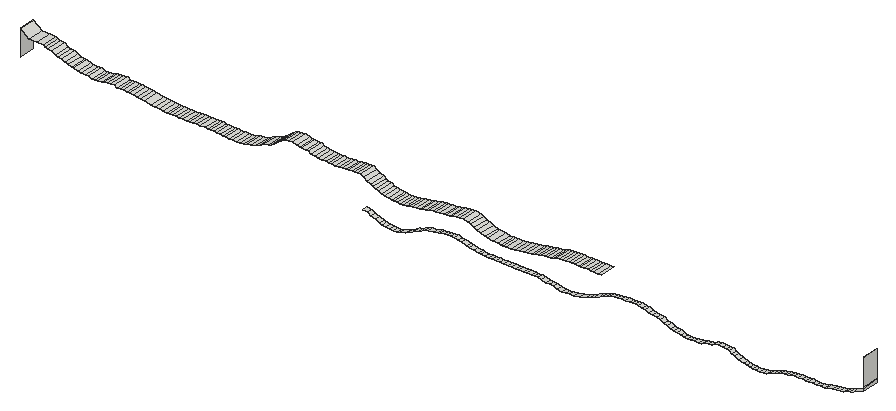
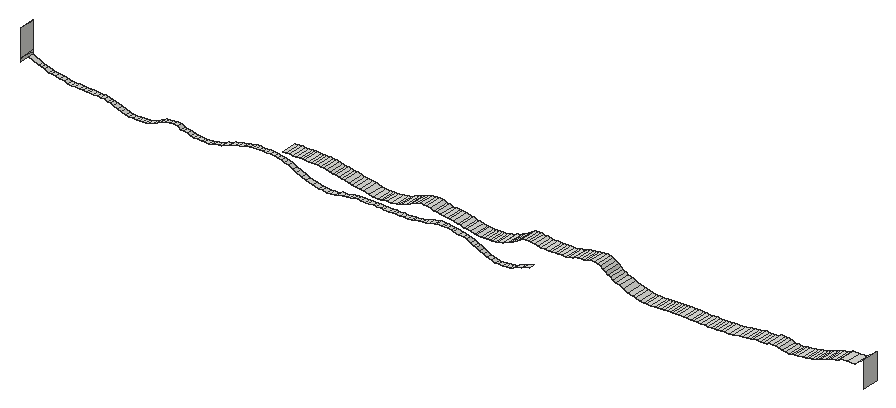
# SketchUp Ruby script. Lengths in inches.
U = 1.inch
M = Sketchup.active_model
def pt(a) = Geom::Point3d.new(a.map { |v| v * U })
def face(e, loops, mat)
  f = e.add_face(loops[0].map { |a| pt(a) })
  loops[1..].each { |l| e.add_face(l.map { |a| pt(a) }).erase! }
  f.material = f.back_material = mat if mat
  f
end
# faces: each face lists its corners as indices into pts; further lists are holes
def faces(e, pts, list, mat = nil) = list.each { |f| face(e, (f[0].is_a?(Array) ? f : [f]).map { |l| l.map { |i| pts[i] } }, mat) }
# xy, xz, yz: faces in a plane at the given z, y or x. An outline is a flat list of corners, or four numbers for a rectangle; further outlines are holes
def ring(l) = l.size == 4 ? [[l[0], l[1]], [l[2], l[1]], [l[2], l[3]], [l[0], l[3]]] : l.each_slice(2).to_a
def flat(e, list, mat, &to3) = list.each { |f| face(e, (f[0].is_a?(Array) ? f : [f]).map { |l| ring(l).map { |u, v| to3.(u, v) } }, mat) }
def xy(e, z, list, mat = nil) = flat(e, list, mat) { |x, y| [x, y, z] }
def xz(e, y, list, mat = nil) = flat(e, list, mat) { |x, z| [x, y, z] }
def yz(e, x, list, mat = nil) = flat(e, list, mat) { |y, z| [x, y, z] }
def lines(e, pts, list) = list.each { |a, b| e.add_line(pt(pts[a]), pt(pts[b])) }
# prism: a flat outline (further loops are holes) pulled along v
def prism(e, loops, v, mat = nil)
  f = face(e, loops, mat); d = Geom::Vector3d.new(v.map { |x| x * U })
  f.pushpull(f.normal.samedirection?(d) ? d.length : -d.length)
end
def box(e, o, s, mat = nil) = prism(e, [[o, [o[0] + s[0], o[1], o[2]], [o[0] + s[0], o[1] + s[1], o[2]], [o[0], o[1] + s[1], o[2]]]], [0, 0, s[2]], mat)
def at(x, y, z, deg = 0) = Geom::Transformation.translation(pt([x, y, z])) * Geom::Transformation.rotation(ORIGIN, Z_AXIS, deg.degrees)
def axes(o, x, y, z) = Geom::Transformation.new([*x, 0, *y, 0, *z, 0, *pt(o).to_a, 1])
def part(name) = M.definitions.add(name)
# library, detail: a bought-in or finely detailed component or shape, given as its bounding box
def library(name, o, s) = part(name).tap { |d| box(d.entities, o, s) }
def detail(e, o, s) = box(e.add_group.entities, o, s)
def put(e, d, t, mat = nil) = e.add_instance(d, t).tap { |i| i.material = mat if mat }
def group(e, t, mat = nil) = e.add_group.tap { |g| g.transformation = t; g.material = mat if mat }.entities
root = M.entities
xy(root,238.18,[[376.03,2401.37,376.71,2402.3]])
xy(root,238.62,[[342.56,2401.37,343.33,2402.3],[343.33,2401.37,343.96,2402.3],[343.96,2401.37,344.72,2402.3],[344.72,2401.37,345.34,2402.3],[345.34,2401.37,346.19,2402.3],
  [346.19,2401.37,346.83,2402.3],[346.83,2401.37,347.45,2402.3]])
xy(root,238.625,[[341.14,2401.37,342,2402.3]])
xy(root,238.89,[[396.95,2401.37,397.63,2402.3]])
xy(root,238.9,[[398.39,2401.37,399.01,2402.3],[399.01,2401.37,399.78,2402.3]])
xy(root,240.43,[[365.23,2401.37,365.8,2402.3]])
xy(root,241.68,[[283.28,2401.37,283.87,2404.3]])
xy(root,241.75,[[285.63,2401.37,286.5,2404.3],[286.5,2401.37,287.12,2404.3],[287.12,2401.37,287.63,2404.3]])
xy(root,243.05,[[358.29,2401.37,358.97,2404.3]])
xy(root,243.07,[[356.4375,2401.37,357.02,2404.3]])
xy(root,243.09,[[353.125,2401.37,353.65,2404.3],[353.65,2401.37,354.17,2404.3],[354.17,2401.37,354.83,2404.3],[354.83,2401.37,355.28,2404.3]])
yz(root,252.84,[[2401.37,241.52,2404.3,246.2]])
yz(root,406.85,[[2401.37,240.89,2401.37,241.29,2404.3,241.52,2404.3,240.89],[2401.37,241.29,2404.3,241.52,2401.37,241.52],[2401.37,241.52,2401.37,246.27,2402.0625,246.36,2404.3,246.43,2404.3,241.52],[2401.37,246.27,2401.37,246.43,2404.3,246.43,2402.0625,246.36]])
p = [[319.64,2401.37,237.11],[319.64,2402.3,237.11],[320.4,2402.3,237.04],[320.4,2401.37,237.04],[321.09,2402.3,237.01],[321.09,2401.37,237.01],
  [321.7,2402.3,236.98],[321.7,2401.37,236.98],[322.38,2402.3,237.22],[322.38,2401.37,237.22],[318.95,2401.37,237.2],[318.95,2402.3,237.2],
  [318.42,2401.37,237.33],[318.42,2402.3,237.33],[323.23,2402.3,237.43],[323.23,2401.37,237.43],[317.75,2401.37,237.68],[317.75,2402.3,237.68],
  [323.85,2402.3,237.74],[323.85,2401.37,237.74],[386.68,2401.37,237.45],[386.68,2402.3,237.45],[387.25,2402.3,237.42],[387.25,2401.37,237.42],
  [387.98,2402.3,237.4],[387.98,2401.37,237.4],[388.66,2402.3,237.47],[388.66,2401.37,237.47],[385.49,2401.37,237.59],[385.49,2402.3,237.59],
  [386.09,2402.3,237.51],[386.09,2401.37,237.51],[389.26,2402.3,237.5625],[389.26,2401.37,237.5625],[384.95,2401.37,237.71],[384.95,2402.3,237.71],
  [389.95,2402.3,237.84],[389.95,2401.37,237.84],[316.8125,2401.37,237.96],[316.8125,2402.3,237.96],[324.55,2402.3,238.02],[324.55,2401.37,238.02],
  [351.69,2401.37,237.79],[351.69,2402.3,237.79],[352.4,2402.3,237.74],[352.4,2401.37,237.74],[353.27,2402.3,237.87],[353.27,2401.37,237.87],
  [384.12,2401.37,238],[384.12,2402.3,238],[350.92,2401.37,237.86],[350.92,2402.3,237.86],[390.63,2402.3,238.08],[390.63,2401.37,238.08],
  [350.29,2401.37,238.15],[350.29,2402.3,238.15],[353.92,2402.3,237.88],[353.92,2401.37,237.88],[355.04,2402.3,238.14],[355.04,2401.37,238.14],
  [316.25,2401.37,238.28],[316.25,2402.3,238.28],[324.99,2402.3,238.375],[324.99,2401.37,238.375],[383.41,2401.37,238.33],[383.41,2402.3,238.33],
  [349.52,2401.37,238.19],[349.52,2402.3,238.19],[356.26,2402.3,238.46],[356.26,2401.37,238.46],[374.01,2401.37,238.19],[374.01,2402.3,238.19],
  [374.83,2402.3,238.15],[374.83,2401.37,238.15],[375.36,2402.3,238.11],[375.36,2401.37,238.11],[376.03,2402.3,238.18],[376.03,2401.37,238.18],
  [391.32,2402.3,238.33],[391.32,2401.37,238.33],[348.9,2401.37,238.25],[348.9,2402.3,238.25],[373.4375,2401.37,238.26],[373.4375,2402.3,238.26],
  [376.71,2401.37,238.18],[376.71,2402.3,238.18],[377.39,2402.3,238.27],[377.39,2401.37,238.27],[315.47,2401.37,238.43],[315.47,2402.3,238.43],
  [348.14,2401.37,238.45],[348.14,2402.3,238.45],[372.87,2401.37,238.48],[372.87,2402.3,238.48],[377.91,2402.3,238.55],[377.91,2401.37,238.55],
  [382.86,2401.37,238.57],[382.86,2402.3,238.57],[391.85,2402.3,238.51],[391.85,2401.37,238.51],[325.55,2402.3,238.51],[325.55,2401.37,238.51],
  [326.1875,2402.3,238.76],[326.1875,2401.37,238.76],[347.45,2401.37,238.62],[347.45,2402.3,238.62],[357.01,2402.3,238.72],[357.01,2401.37,238.72],
  [372.21,2401.37,238.56],[372.21,2402.3,238.56],[378.57,2402.3,238.61],[378.57,2401.37,238.61],[392.42,2402.3,238.6],[392.42,2401.37,238.6],
  [338.38,2401.37,238.66],[338.38,2402.3,238.66],[339.05,2402.3,238.65],[339.05,2401.37,238.65],[339.83,2402.3,238.64],[339.83,2401.37,238.64],
  [340.45,2402.3,238.63],[340.45,2401.37,238.63],[341.14,2402.3,238.625],[341.14,2401.37,238.625],[342,2401.37,238.625],[342,2402.3,238.625],
  [342.56,2402.3,238.62],[342.56,2401.37,238.62],[371.64,2401.37,238.67],[371.64,2402.3,238.67],[379.16,2402.3,238.66],[379.16,2401.37,238.66],
  [382.36,2401.37,238.86],[382.36,2402.3,238.86],[393.08,2402.3,238.74],[393.08,2401.37,238.74],[336.54,2401.37,238.78],[336.54,2402.3,238.78],
  [337.02,2402.3,238.73],[337.02,2401.37,238.73],[337.69,2402.3,238.6875],[337.69,2401.37,238.6875],[357.89,2402.3,239.08],[357.89,2401.37,239.08],
  [371.12,2401.37,239.01],[371.12,2402.3,239.01],[379.73,2402.3,239.04],[379.73,2401.37,239.04],[393.66,2402.3,238.8],[393.66,2401.37,238.8],
  [326.83,2402.3,239.12],[326.83,2401.37,239.12],[335.66,2401.37,238.93],[335.66,2402.3,238.93],[394.23,2402.3,238.83],[394.23,2401.37,238.83],
  [394.97,2402.3,238.86],[394.97,2401.37,238.86],[334.89,2401.37,239.07],[334.89,2402.3,239.07],[381.84,2401.37,238.96],[381.84,2402.3,238.96],
  [395.73,2402.3,238.875],[395.73,2401.37,238.875],[396.27,2402.3,238.88],[396.27,2401.37,238.88],[396.95,2402.3,238.89],[396.95,2401.37,238.89],
  [397.63,2401.37,238.89],[397.63,2402.3,238.89],[398.39,2402.3,238.9],[398.39,2401.37,238.9],[399.78,2401.37,238.9],[399.78,2402.3,238.9],
  [400.41,2402.3,239.15],[400.41,2401.37,239.15],[370.4375,2401.37,239.18],[370.4375,2402.3,239.18],[380.47,2402.3,239.125],[380.47,2401.37,239.125],
  [381.15,2402.3,239.02],[381.15,2401.37,239.02],[327.41,2402.3,239.22],[327.41,2401.37,239.22],[334.34,2401.37,239.16],[334.34,2402.3,239.16],
  [358.68,2402.3,239.375],[358.68,2401.37,239.375],[328.41,2402.3,239.31],[328.41,2401.37,239.31],[333.49,2401.37,239.44],[333.49,2402.3,239.44],
  [369.8125,2401.37,239.5],[369.8125,2402.3,239.5],[401.18,2402.3,239.28],[401.18,2401.37,239.28],[329.22,2402.3,239.54],[329.22,2401.37,239.54],
  [401.98,2402.3,239.42],[401.98,2401.37,239.42],[332.82,2401.37,239.56],[332.82,2402.3,239.56],[359.42,2402.3,239.75],[359.42,2401.37,239.75],
  [402.7,2402.3,239.49],[402.7,2401.37,239.49],[329.71,2402.3,239.6],[329.71,2401.37,239.6],[369.05,2401.37,239.65],[369.05,2402.3,239.65],
  [403.25,2402.3,239.53],[403.25,2401.37,239.53],[403.9375,2402.3,239.81],[403.9375,2401.37,239.81],[330.33,2402.3,239.65],[330.33,2401.37,239.65],
  [330.92,2402.3,239.69],[330.92,2401.37,239.69],[332.21,2401.37,239.72],[332.21,2402.3,239.72],[331.48,2402.3,239.7],[331.48,2401.37,239.7],
  [360.07,2402.3,239.97],[360.07,2401.37,239.97],[368.4375,2401.37,239.8],[368.4375,2402.3,239.8],[367.68,2401.37,239.96],[367.68,2402.3,239.96],
  [404.46,2402.3,239.96],[404.46,2401.37,239.96],[360.69,2402.3,240.17],[360.69,2401.37,240.17],[367.03,2401.37,240.23],[367.03,2402.3,240.23],
  [405.02,2402.3,240.1],[405.02,2401.37,240.1],[406.85,2402.3,240.89],[406.85,2401.37,240.89],[361.37,2402.3,240.27],[361.37,2401.37,240.27],
  [366.45,2401.37,240.27],[366.45,2402.3,240.27],[362.05,2402.3,240.33],[362.05,2401.37,240.33],[362.74,2402.3,240.37],[362.74,2401.37,240.37],
  [365.8,2401.37,240.43],[365.8,2402.3,240.43],[363.43,2402.3,240.4],[363.43,2401.37,240.4],[364.125,2402.3,240.41],[364.125,2401.37,240.41],
  [364.65,2402.3,240.42],[364.65,2401.37,240.42],[365.23,2402.3,240.43],[365.23,2401.37,240.43],[289.26,2404.3,241.57],[289.8,2404.3,241.53],
  [289.8,2401.37,241.53],[289.26,2401.37,241.57],[290.42,2404.3,241.51],[290.42,2401.37,241.51],[290.97,2404.3,241.49],[290.97,2401.37,241.49],
  [291.67,2404.3,241.48],[291.67,2401.37,241.48],[292.33,2404.3,241.47],[292.33,2401.37,241.47],[292.9,2404.3,241.46],[292.9,2401.37,241.46],
  [293.61,2404.3,241.6],[293.61,2401.37,241.6],[339.98,2404.3,241.56],[340.58,2404.3,241.51],[340.58,2401.37,241.51],[339.98,2401.37,241.56],
  [341.03,2404.3,241.48],[341.03,2401.37,241.48],[341.55,2404.3,241.46],[341.55,2401.37,241.46],[342.42,2404.3,241.51],[342.42,2401.37,241.51],
  [343.14,2404.3,241.59],[343.14,2401.37,241.59],[288.65,2404.3,241.66],[288.65,2401.37,241.66],[294.34,2404.3,241.85],[294.34,2401.37,241.85],
  [338.16,2404.3,241.78],[339.21,2404.3,241.63],[339.21,2401.37,241.63],[338.16,2401.37,241.78],[344.08,2404.3,241.82],[344.08,2401.37,241.82],
  [279.62,2404.3,241.75],[280.07,2404.3,241.74],[280.07,2401.37,241.74],[279.62,2401.37,241.75],[280.62,2404.3,241.72],[280.62,2401.37,241.72],
  [281.25,2404.3,241.71],[281.25,2401.37,241.71],[281.88,2404.3,241.7],[281.88,2401.37,241.7],[282.61,2404.3,241.69],[282.61,2401.37,241.69],
  [283.28,2404.3,241.68],[283.28,2401.37,241.68],[283.87,2404.3,241.68],[284.36,2404.3,241.67],[284.36,2401.37,241.67],[283.87,2401.37,241.68],
  [285.0625,2404.3,241.74],[285.0625,2401.37,241.74],[285.63,2404.3,241.75],[285.63,2401.37,241.75],[287.63,2404.3,241.75],[288.12,2404.3,241.67],
  [288.12,2401.37,241.67],[287.63,2401.37,241.75],[277.43,2404.3,241.89],[278.25,2404.3,241.83],[278.25,2401.37,241.83],[277.43,2401.37,241.89],
  [278.85,2404.3,241.78],[278.85,2401.37,241.78],[295.01,2404.3,241.91],[295.01,2401.37,241.91],[320.64,2404.3,241.89],[321.1,2404.3,241.85],
  [321.1,2401.37,241.85],[320.64,2401.37,241.89],[321.62,2404.3,241.8125],[321.62,2401.37,241.8125],[322.13,2404.3,241.79],[322.13,2401.37,241.79],
  [322.71,2404.3,241.78],[322.71,2401.37,241.78],[323.38,2404.3,241.91],[323.38,2401.37,241.91],[337.67,2404.3,241.89],[337.67,2401.37,241.89],
  [344.86,2404.3,241.87],[344.86,2401.37,241.87],[276.66,2404.3,241.96],[276.66,2401.37,241.96],[295.91,2404.3,242.1],[295.91,2401.37,242.1],
  [320.08,2404.3,241.96],[320.08,2401.37,241.96],[323.85,2404.3,241.93],[323.85,2401.37,241.93],[324.52,2404.3,242.09],[324.52,2401.37,242.09],
  [337.03,2404.3,242.14],[337.03,2401.37,242.14],[345.625,2404.3,241.98],[345.625,2401.37,241.98],[275.49,2404.3,242.24],[275.49,2401.37,242.24],
  [319.4,2404.3,242.11],[319.4,2401.37,242.11],[346.24,2404.3,242.02],[346.24,2401.37,242.02],[346.89,2404.3,242.19],[346.89,2401.37,242.19],
  [296.68,2404.3,242.46],[296.68,2401.37,242.46],[318.8,2404.3,242.21],[318.8,2401.37,242.21],[325.29,2404.3,242.2],[325.29,2401.37,242.2],
  [336.27,2404.3,242.39],[336.27,2401.37,242.39],[274.82,2404.3,242.34],[274.82,2401.37,242.34],[318.29,2404.3,242.51],[318.29,2401.37,242.51],
  [325.79,2404.3,242.24],[325.79,2401.37,242.24],[326.4,2404.3,242.42],[326.4,2401.37,242.42],[347.59,2404.3,242.38],[347.59,2401.37,242.38],
  [274.16,2404.3,242.38],[274.16,2401.37,242.38],[273.5,2404.3,242.48],[273.5,2401.37,242.48],[326.95,2404.3,242.47],[326.95,2401.37,242.47],
  [335.65,2404.3,242.65],[335.65,2401.37,242.65],[348.08,2404.3,242.4375],[348.08,2401.37,242.4375],[348.6,2404.3,242.48],[348.6,2401.37,242.48],
  [265.32,2404.3,242.68],[265.99,2404.3,242.51],[265.99,2401.37,242.51],[265.32,2401.37,242.68],[266.51,2404.3,242.46],[266.51,2401.37,242.46],
  [267.05,2404.3,242.58],[267.05,2401.37,242.58],[272.86,2404.3,242.57],[272.86,2401.37,242.57],[297.38,2404.3,242.78],[297.38,2401.37,242.78],
  [317.7,2404.3,242.68],[317.7,2401.37,242.68],[327.7,2404.3,242.71],[327.7,2401.37,242.71],[349.26,2404.3,242.58],[349.26,2401.37,242.58],
  [267.68,2404.3,242.57],[267.68,2401.37,242.57],[268.31,2404.3,242.81],[268.31,2401.37,242.81],[270.08,2404.3,242.92],[270.51,2404.3,242.625],
  [270.51,2401.37,242.625],[270.08,2401.37,242.92],[271.12,2404.3,242.65],[271.12,2401.37,242.65],[271.67,2404.3,242.62],[271.67,2401.37,242.62],
  [272.3,2404.3,242.58],[272.3,2401.37,242.58],[335.1,2404.3,242.9375],[335.1,2401.37,242.9375],[349.79,2404.3,242.61],[349.79,2401.37,242.61],
  [350.375,2404.3,242.77],[350.375,2401.37,242.77],[263.97,2404.3,242.78],[264.78,2404.3,242.73],[264.78,2401.37,242.73],[263.97,2401.37,242.78],
  [317.2,2404.3,242.875],[317.2,2401.37,242.875],[328.34,2404.3,242.78],[328.34,2401.37,242.78],[262.67,2404.3,243.06],[263.39,2404.3,242.85],
  [263.39,2401.37,242.85],[262.67,2401.37,243.06],[268.88,2404.3,242.86],[268.88,2401.37,242.86],[298.15,2404.3,242.97],[298.15,2401.37,242.97],
  [328.82,2404.3,242.82],[328.82,2401.37,242.82],[329.51,2404.3,242.85],[329.51,2401.37,242.85],[350.83,2404.3,242.95],[350.83,2401.37,242.95],
  [269.44,2404.3,242.89],[269.44,2401.37,242.89],[316.81,2404.3,243.09],[316.81,2401.37,243.09],[330.21,2404.3,242.87],[330.21,2401.37,242.87],
  [330.76,2404.3,243.02],[330.76,2401.37,243.02],[334.53,2404.3,243.14],[334.53,2401.37,243.14],[298.68,2404.3,243.23],[298.68,2401.37,243.23],
  [331.38,2404.3,243.05],[331.38,2401.37,243.05],[351.39,2404.3,243.01],[351.39,2401.37,243.01],[351.9,2404.3,243.05],[351.9,2401.37,243.05],
  [352.47,2404.3,243.08],[352.47,2401.37,243.08],[261.6,2404.3,243.3],[262.1875,2404.3,243.14],[262.1875,2401.37,243.14],[261.6,2401.37,243.3],
  [316.2,2404.3,243.43],[316.2,2401.37,243.43],[331.93,2404.3,243.29],[331.93,2401.37,243.29],[333.76,2404.3,243.42],[333.76,2401.37,243.42],
  [353.125,2404.3,243.09],[353.125,2401.37,243.09],[355.28,2404.3,243.09],[355.85,2404.3,243.08],[355.85,2401.37,243.08],[355.28,2401.37,243.09],
  [356.4375,2404.3,243.07],[356.4375,2401.37,243.07],[357.02,2404.3,243.07],[357.68,2404.3,243.0625],[357.68,2401.37,243.0625],[357.02,2401.37,243.07],
  [358.29,2404.3,243.05],[358.29,2401.37,243.05],[299.08,2404.3,243.48],[299.08,2401.37,243.48],[260.96,2404.3,243.48],[260.96,2401.37,243.48],
  [332.61,2404.3,243.35],[332.61,2401.37,243.35],[315.66,2404.3,243.8],[315.66,2401.37,243.8],[333.16,2404.3,243.39],[333.16,2401.37,243.39],
  [260.44,2404.3,243.79],[260.44,2401.37,243.79],[299.6,2404.3,243.72],[299.6,2401.37,243.72],[299.9375,2404.3,244.12],[299.9375,2401.37,244.12],
  [259.78,2404.3,243.95],[259.78,2401.37,243.95],[315.06,2404.3,244.18],[315.06,2401.37,244.18],[259.26,2404.3,244.11],[259.26,2401.37,244.11],
  [307.88,2404.3,243.99],[308.6,2404.3,243.95],[308.6,2401.37,243.95],[307.88,2401.37,243.99],[309.1,2404.3,243.93],[309.1,2401.37,243.93],
  [309.79,2404.3,243.91],[309.79,2401.37,243.91],[310.36,2404.3,243.89],[310.36,2401.37,243.89],[311.06,2404.3,243.88],[311.06,2401.37,243.88],
  [311.71,2404.3,243.94],[311.71,2401.37,243.94],[312.35,2404.3,243.95],[312.35,2401.37,243.95],[312.91,2404.3,244.1],[312.91,2401.37,244.1],
  [306.7,2404.3,244.11],[307.26,2404.3,244.04],[307.26,2401.37,244.04],[306.7,2401.37,244.11],[258.59,2404.3,244.41],[258.59,2401.37,244.41],
  [300.41,2404.3,244.39],[300.41,2401.37,244.39],[305.95,2404.3,244.25],[305.95,2401.37,244.25],[313.54,2404.3,244.13],[313.54,2401.37,244.13],
  [314.02,2404.3,244.15],[314.02,2401.37,244.15],[314.54,2404.3,244.17],[314.54,2401.37,244.17],[305.49,2404.3,244.51],[305.49,2401.37,244.51],
  [257.83,2404.3,244.54],[257.83,2401.37,244.54],[300.89,2404.3,244.73],[300.89,2401.37,244.73],[257.27,2404.3,244.61],[257.27,2401.37,244.61],
  [304.34,2404.3,244.67],[304.95,2404.3,244.55],[304.95,2401.37,244.55],[304.34,2401.37,244.67],[257.05,2404.3,244.92],[257.05,2401.37,244.92],
  [301.375,2404.3,244.87],[301.375,2401.37,244.87],[303.29,2404.3,244.81],[303.86,2404.3,244.7],[303.86,2401.37,244.7],[303.29,2401.37,244.81],
  [302.64,2404.3,245.01],[302.64,2401.37,245.01],[254.41,2404.3,244.96],[255.8,2404.3,244.9375],[255.8,2401.37,244.9375],[254.41,2401.37,244.96],
  [301.96,2404.3,244.95],[301.96,2401.37,244.95],[252.84,2404.3,246.2],[252.84,2401.37,246.2]]
faces(root,p,[[0,1,2,3],[3,2,4,5],[5,4,6,7],[7,6,8,9],[10,11,1,0],[12,13,11,10],[9,8,14,15],[16,17,13,12],
  [15,14,18,19],[20,21,22,23],[23,22,24,25],[25,24,26,27],[28,29,30,31],[31,30,21,20],[27,26,32,33],[34,35,29,28],
  [33,32,36,37],[38,39,17,16],[19,18,40,41],[42,43,44,45],[45,44,46,47],[48,49,35,34],[50,51,43,42],[37,36,52,53],
  [54,55,51,50],[47,46,56,57],[57,56,58,59],[60,61,39,38],[41,40,62,63],[64,65,49,48],[66,67,55,54],[59,58,68,69],
  [70,71,72,73],[73,72,74,75],[75,74,76,77],[53,52,78,79],[80,81,67,66],[82,83,71,70],[84,85,86,87],[88,89,61,60],
  [90,91,81,80],[92,93,83,82],[87,86,94,95],[96,97,65,64],[79,78,98,99],[63,62,100,101],[101,100,102,103],[104,105,91,90],
  [69,68,106,107],[108,109,93,92],[95,94,110,111],[99,98,112,113],[114,115,116,117],[117,116,118,119],[119,118,120,121],[121,120,122,123],
  [124,125,126,127],[128,129,109,108],[111,110,130,131],[132,133,97,96],[113,112,134,135],[136,137,138,139],[139,138,140,141],[141,140,115,114],
  [107,106,142,143],[144,145,129,128],[131,130,146,147],[135,134,148,149],[103,102,150,151],[152,153,137,136],[149,148,154,155],[155,154,156,157],
  [158,159,153,152],[160,161,133,132],[157,156,162,163],[163,162,164,165],[165,164,166,167],[168,169,170,171],[172,173,174,175],[176,177,145,144],
  [147,146,178,179],[179,178,180,181],[181,180,161,160],[151,150,182,183],[184,185,159,158],[143,142,186,187],[183,182,188,189],[190,191,185,184],
  [192,193,177,176],[175,174,194,195],[189,188,196,197],[195,194,198,199],[200,201,191,190],[187,186,202,203],[199,198,204,205],[197,196,206,207],
  [208,209,193,192],[205,204,210,211],[211,210,212,213],[207,206,214,215],[215,214,216,217],[218,219,201,200],[217,216,220,221],[221,220,219,218],
  [203,202,222,223],[224,225,209,208],[226,227,225,224],[213,212,228,229],[223,222,230,231],[232,233,227,226],[229,228,234,235],[235,234,236,237],
  [231,230,238,239],[240,241,233,232],[239,238,242,243],[243,242,244,245],[246,247,241,240],[245,244,248,249],[249,248,250,251],[251,250,252,253],
  [253,252,254,255],[256,257,258,259],[257,260,261,258],[260,262,263,261],[262,264,265,263],[264,266,267,265],[266,268,269,267],[268,270,271,269],
  [272,273,274,275],[273,276,277,274],[276,278,279,277],[278,280,281,279],[280,282,283,281],[284,256,259,285],[270,286,287,271],[288,289,290,291],
  [289,272,275,290],[282,292,293,283],[294,295,296,297],[295,298,299,296],[298,300,301,299],[300,302,303,301],[302,304,305,303],[304,306,307,305],
  [308,309,310,311],[309,312,313,310],[312,314,315,313],[316,317,318,319],[317,284,285,318],[320,321,322,323],[321,324,325,322],[324,294,297,325],
  [286,326,327,287],[328,329,330,331],[329,332,333,330],[332,334,335,333],[334,336,337,335],[336,338,339,337],[340,288,291,341],[292,342,343,293],
  [344,320,323,345],[326,346,347,327],[348,328,331,349],[338,350,351,339],[350,352,353,351],[354,340,341,355],[342,356,357,343],[358,344,345,359],
  [360,348,349,361],[356,362,363,357],[362,364,365,363],[346,366,367,347],[368,360,361,369],[352,370,371,353],[372,354,355,373],[374,358,359,375],
  [376,368,369,377],[370,378,379,371],[378,380,381,379],[364,382,383,365],[384,374,375,385],[386,384,385,387],[380,388,389,381],[390,372,373,391],
  [382,392,393,383],[392,394,395,393],[396,397,398,399],[397,400,401,398],[400,402,403,401],[404,386,387,405],[366,406,407,367],[408,376,377,409],
  [388,410,411,389],[394,412,413,395],[402,414,415,403],[414,416,417,415],[418,419,420,421],[419,422,423,420],[422,424,425,423],[424,426,427,425],
  [426,404,405,427],[428,390,391,429],[412,430,431,413],[430,432,433,431],[434,435,436,437],[435,396,399,436],[438,408,409,439],[410,440,441,411],
  [442,443,444,445],[443,434,437,444],[416,446,447,417],[406,448,449,407],[440,450,451,441],[450,452,453,451],[432,454,455,433],[446,456,457,447],
  [456,418,421,457],[458,438,439,459],[452,460,461,453],[460,462,463,461],[464,428,429,465],[448,466,467,449],[462,468,469,463],[454,470,471,455],
  [470,472,473,471],[472,474,475,473],[476,477,478,479],[477,442,445,478],[480,458,459,481],[468,482,483,469],[484,464,465,485],[474,486,487,475],
  [488,489,490,491],[489,492,493,490],[494,495,496,497],[495,498,499,496],[466,500,501,467],[502,476,479,503],[482,504,505,483],[506,480,481,507],
  [504,508,509,505],[508,484,485,509],[510,502,503,511],[500,512,513,501],[512,514,515,513],[516,510,511,517],[518,506,507,519],[520,516,517,521],
  [522,523,524,525],[523,526,527,524],[526,528,529,527],[528,530,531,529],[530,532,533,531],[532,534,535,533],[534,536,537,535],[536,538,539,537],
  [540,541,542,543],[541,522,525,542],[544,520,521,545],[514,546,547,515],[548,540,543,549],[538,550,551,539],[550,552,553,551],[552,554,555,553],
  [554,518,519,555],[556,548,549,557],[558,544,545,559],[546,560,561,547],[562,558,559,563],[564,565,566,567],[565,556,557,566],[568,562,563,569],
  [560,570,571,561],[572,573,574,575],[573,564,567,574],[576,572,575,577],[578,579,580,581],[579,568,569,580],[570,582,583,571],[582,576,577,583],
  [584,578,581,585]])
